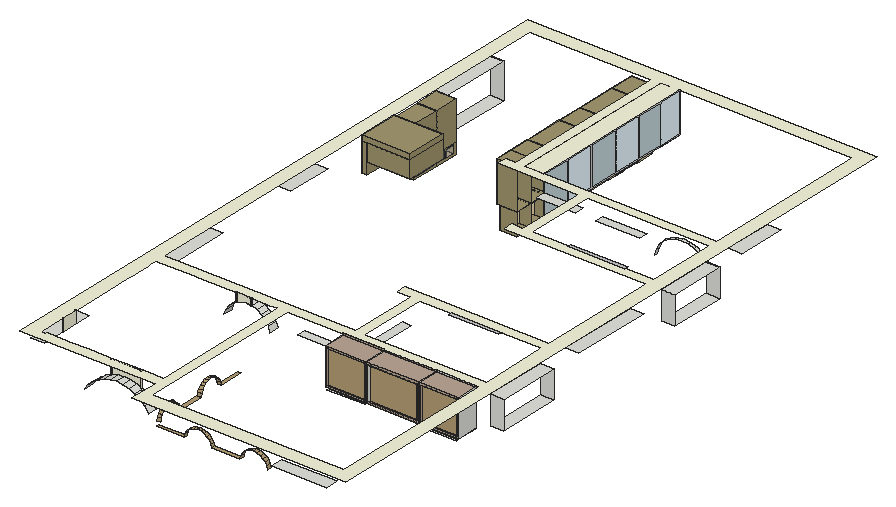
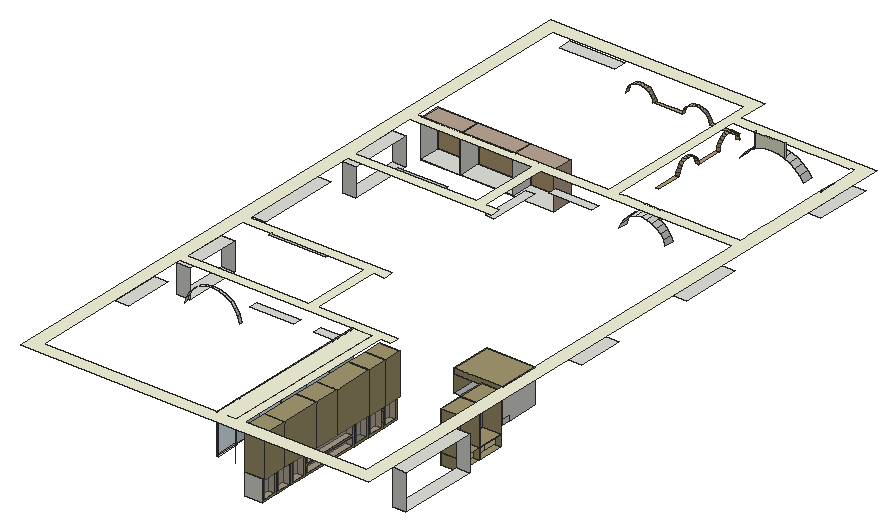
# SketchUp Ruby script. Lengths in inches.
U = 1.inch
M = Sketchup.active_model
def pt(a) = Geom::Point3d.new(a.map { |v| v * U })
def face(e, loops, mat)
  f = e.add_face(loops[0].map { |a| pt(a) })
  loops[1..].each { |l| e.add_face(l.map { |a| pt(a) }).erase! }
  f.material = f.back_material = mat if mat
  f
end
# faces: each face lists its corners as indices into pts; further lists are holes
def faces(e, pts, list, mat = nil) = list.each { |f| face(e, (f[0].is_a?(Array) ? f : [f]).map { |l| l.map { |i| pts[i] } }, mat) }
# xy, xz, yz: faces in a plane at the given z, y or x. An outline is a flat list of corners, or four numbers for a rectangle; further outlines are holes
def ring(l) = l.size == 4 ? [[l[0], l[1]], [l[2], l[1]], [l[2], l[3]], [l[0], l[3]]] : l.each_slice(2).to_a
def flat(e, list, mat, &to3) = list.each { |f| face(e, (f[0].is_a?(Array) ? f : [f]).map { |l| ring(l).map { |u, v| to3.(u, v) } }, mat) }
def xy(e, z, list, mat = nil) = flat(e, list, mat) { |x, y| [x, y, z] }
def xz(e, y, list, mat = nil) = flat(e, list, mat) { |x, z| [x, y, z] }
def yz(e, x, list, mat = nil) = flat(e, list, mat) { |y, z| [x, y, z] }
def lines(e, pts, list) = list.each { |a, b| e.add_line(pt(pts[a]), pt(pts[b])) }
# prism: a flat outline (further loops are holes) pulled along v
def prism(e, loops, v, mat = nil)
  f = face(e, loops, mat); d = Geom::Vector3d.new(v.map { |x| x * U })
  f.pushpull(f.normal.samedirection?(d) ? d.length : -d.length)
end
def box(e, o, s, mat = nil) = prism(e, [[o, [o[0] + s[0], o[1], o[2]], [o[0] + s[0], o[1] + s[1], o[2]], [o[0], o[1] + s[1], o[2]]]], [0, 0, s[2]], mat)
def at(x, y, z, deg = 0) = Geom::Transformation.translation(pt([x, y, z])) * Geom::Transformation.rotation(ORIGIN, Z_AXIS, deg.degrees)
def axes(o, x, y, z) = Geom::Transformation.new([*x, 0, *y, 0, *z, 0, *pt(o).to_a, 1])
def part(name) = M.definitions.add(name)
# library, detail: a bought-in or finely detailed component or shape, given as its bounding box
def library(name, o, s) = part(name).tap { |d| box(d.entities, o, s) }
def detail(e, o, s) = box(e.add_group.entities, o, s)
def put(e, d, t, mat = nil) = e.add_instance(d, t).tap { |i| i.material = mat if mat }
def group(e, t, mat = nil) = e.add_group.tap { |g| g.transformation = t; g.material = mat if mat }.entities
root = M.entities
M.materials.add("[0034_Wheat]").color = [245, 222, 179]
M.materials.add("[0049_Beige]").color = [245, 245, 220]
M.materials.add("[0093_AliceBlue]").color = [232, 248, 255]
M.materials.add("[0095_LightBlue]").color = [197, 216, 221]
M.materials.add("[0119_RosyBrown]").color = [188, 166, 148]
M.materials.add("[0132_LightGray]").color = [169, 169, 169]
M.materials.add("[Carrera Marble]").color = [207, 207, 207]
M.materials.add("[Ornate Tile 01]").color = [202, 202, 202]
M.materials.add("[Ornate Tile 02]").color = [201, 201, 201]
M.materials.add("[Translucent Glass Gray]").color = [128, 128, 128]
M.materials["[Translucent Glass Gray]"].alpha = 0.5
M.materials.add("[Wallpaper Thin Brown Stripes]").color = [182, 160, 118]
M.materials.add("[Wood Lumber ButtJoined]").color = [164, 152, 112]
xy(root,74.375,[[81.125,330.5,93,342.5],[81.125,342.99,93,354.99],[81.125,355.39,93,367.39],[81.125,367.79,93,409.3],[81.125,409.7,93,421.7],
  [81.125,422.1,93,434.1],[81.125,434.5,93,446.5]],"[Wood Lumber ButtJoined]")
xy(root,75.375,[[81.125,331.5,85.875,341.5],[81.125,343.99,85.875,353.99],[81.125,368.79,85.875,408.3],[81.125,410.7,85.875,420.7],[81.125,423.1,85.875,433.1],
  [81.125,435.5,85.875,445.5]],"[0034_Wheat]")
xy(root,75.375,[[81.125,356.39,85.875,366.39]],"[Wood Lumber ButtJoined]")
xy(root,81.08,[[81.125,368.79,85.875,408.3]],"[0034_Wheat]")
xy(root,81.8125,[[81.125,368.79,85.875,408.3]],"[0034_Wheat]")
xy(root,83.7,[[9,331.5,21.5,350.0625],[9,350.25,21.5,367.1875]],"[Wood Lumber ButtJoined]")
xy(root,84.7,[[12.5625,340.53,21.5,341.09],[12.5625,358.53,21.5,359.02]])
xy(root,84.7,[[12.5625,332.5,21.5,340.53],[12.5625,341.09,21.5,349.0625],[12.5625,351.25,21.5,358.53],[12.5625,359.02,21.5,366.1875]],"[0034_Wheat]")
xy(root,87.5625,[[0,369.625,9,424.25]])
xy(root,88.25,[[81.125,331.5,85.875,341.5],[81.125,343.99,85.875,353.99],[81.125,356.39,85.875,366.39],[81.125,368.79,85.875,408.3],[81.125,410.7,85.875,420.7],
  [81.125,423.1,85.875,433.1],[81.125,435.5,85.875,445.5]],"[0034_Wheat]")
xy(root,89.25,[[81.125,355.39,93,367.39],[81.125,367.79,93,409.3]])
xy(root,89.25,[[81.125,330.5,93,342.5],[81.125,342.99,93,354.99],[81.125,409.7,93,421.7],[81.125,422.1,93,434.1],[81.125,434.5,93,446.5]],"[Wood Lumber ButtJoined]")
xy(root,89.4375,[[79.125,330.5,93,342.84],[79.125,342.99,93,356.99],[79.125,357.2,93,384.45],[79.125,384.7,93,401.95],[79.125,402.1,93,429.35],
  [79.125,429.5,93,446.5]],"[Wood Lumber ButtJoined]")
xy(root,90.26,[[12.5625,332.5,21.5,340.53],[12.5625,341.09,21.5,349.0625],[12.5625,351.25,21.5,358.53],[12.5625,359.02,21.5,366.1875]],"[0034_Wheat]")
xy(root,91.26,[[9,331.5,21.5,350.0625],[9,350.25,21.5,367.1875]],"[Wood Lumber ButtJoined]")
xy(root,91.5625,[[9,331.5,22.125,350.0625],[9,350.25,22.125,367.1875]],"[Wood Lumber ButtJoined]")
xy(root,92,[[231,135.375,240,178.8125],[231,282.5625,240,321.125]])
xy(root,92.17,[[202.62,111,227.31,112.1875]])
xy(root,92.18,[[111.3125,350.49,112,370.8125],[111.3125,392.31,112,411.67],[111.3125,430.5,112,446.4]])
xy(root,92.2,[[138.21,111,163.85,112.1875]])
xy(root,93.18,[[111.5,330.5,112,350.375],[111.5,371.18,112,392.06],[111.5,411.92,112,430.3]],"[Carrera Marble]")
xy(root,93.41,[[137,111,165.0625,126],[165.15,111,201.29,126],[201.375,111,228.5625,126]])
xy(root,93.5625,[[137,111,165.0625,126],[165.15,111,201.29,126],[201.375,111,228.5625,126]])
xy(root,94.54,[[202.35,111,227.59,112.1875]],"[0119_RosyBrown]")
xy(root,94.64,[[138.08,111,163.98,112.1875]],"[0119_RosyBrown]")
xy(root,94.89,[[166.48,111,199.96,112.1875]],"[0119_RosyBrown]")
xy(root,96.5,[[9,302.05,12.875,330]])
xy(root,101.92,[[99,31.4,101.25,48.4],[99,66.3,101.25,83.1]],"[Wallpaper Thin Brown Stripes]")
xy(root,102.01,[[102.48,9,121.18,11.25],[140.76,9,159.46,11.25]],"[Wallpaper Thin Brown Stripes]")
xy(root,104.75,[[12.875,302.05,42.3125,330]],"[0132_LightGray]")
xy(root,108,[[105.75,126,136,132],[141,137.75,147,172.25],[112,324,138.73,330],[152.79,324,183.21,330]])
xy(root,111.25,[[231,135.375,240,178.8125],[231,200.3125,240,256],[231,282.5625,240,321.125],[231,340.4375,240,373.75]])
xy(root,111.6875,[[188.875,0,226.8125,9]])
xy(root,111.75,[[0,29.375,0,67.375,9.5,67.375,9.5,56.09,9,56.09,9,55.89,9.5,55.89,9.5,45.39,9,45.39,9,45.1875,9.25,45.1875,9.25,29.375],[0,141.25,9,183],[0,241.5625,9,273.5],[0,369.625,9,424.25]])
xy(root,113.91,[[64.01,125.5625,64.21,126]],"[0049_Beige]")
xy(root,116.5,[[9,302.05,12.875,330],[12.875,302.05,42.3125,330]])
xy(root,117.625,[[79.125,330.5,93,342.84],[79.125,342.99,93,356.99],[79.125,357.2,93,384.45],[79.125,384.7,93,401.95],[79.125,402.1,93,429.35],
  [79.125,429.5,93,446.5]],"[Wood Lumber ButtJoined]")
xy(root,117.67,[[166.48,111,199.96,112.1875]],"[0119_RosyBrown]")
xy(root,117.92,[[138.08,111,163.98,112.1875]],"[0119_RosyBrown]")
xy(root,118.02,[[202.35,111,227.59,112.1875]],"[0119_RosyBrown]")
xy(root,118.3125,[[9,331.5,22.125,350.0625],[9,350.25,22.125,367.1875]],"[Wood Lumber ButtJoined]")
xy(root,119,[[137,111,165.0625,126],[165.15,111,201.29,126],[201.375,111,228.5625,126]],"[0119_RosyBrown]")
xy(root,119.5,[[111.5,371.18,112,392.06],[111.5,411.92,112,430.3]])
xy(root,119.5,[[111.5,330.5,112,350.375]],"[Carrera Marble]")
xy(root,120,[[[93,0,240,0,240,456,0,456,0,20,93,20],[9,132,9,447,93,447,93,330,86,330,86,324,141,324,141,276,133.48,276,133.48,270,231,270,231,186,131.5,186,131.5,180,141,180,141,132],[99,9,231,126],[112,330,231,447],[9.25,26,9.25,45.1875,9,45.1875,9,45.39,9.5,45.39,9.5,55.89,9,55.89,9,56.09,9.5,56.09,9.5,71.78,9,71.78,9,71.98,9.5,71.98,9.5,83.1,9,83.1,9,83.3,9.5,83.3,9.5,102.55,9,102.55,9,102.75,9.5,102.75,9.5,118.43,9,118.43,9,125.5625,30.5625,125.5625,30.5625,126,30.76,126,30.76,125.5625,42.33,125.5625,42.33,126,42.53,126,42.53,125.5625,64.01,125.5625,64.01,126,64.21,126,64.21,125.5625,74.41,125.5625,74.41,126,74.6,126,74.6,125.5625,88.16,125.5625,88.16,126,93,126,93,26.8125,78.0625,26.8125,78.0625,26,77.86,26,77.86,26.8125,57.8,26.8125,57.8,26,57.6,26,57.6,26.8125,41.25,26.8125,41.25,26,41.05,26,41.05,26.8125,29.25,26.8125,29.25,26,29.05,26,29.05,26.8125,12.5625,26.8125,12.5625,26],[147,132,231,180],[147,276,231,324]]],"[0049_Beige]")
xy(root,120,[[168.74,177.6875,203.125,180]],"[Ornate Tile 01]")
xy(root,120,[[171.75,276,211.1875,278.4375]],"[Ornate Tile 02]")
xy(root,120,[[9,302.05,42.3125,330]],"[Wood Lumber ButtJoined]")
xz(root,26,[[57.6,110.54,57.8,110.63,57.8,110.54]])
xz(root,26,[[78.0625,109.3125,77.86,109.4,77.86,120,78.0625,120],[57.6,110.54,57.6,120,57.8,120,57.8,110.63]],"[0049_Beige]")
xz(root,26.8125,[[77.86,109.4,75,110.68,70.79,111.76,66.46,112.125,62.125,111.76,57.92,110.68,57.8,110.63,57.8,120,77.86,120]],"[0049_Beige]")
xz(root,45.1875,[[9,111.75,9.25,120]],"[0049_Beige]")
xz(root,45.39,[[9,111.75,9.5,120]],"[0049_Beige]")
xz(root,55.89,[[9,111.75,9.5,120]],"[0049_Beige]")
xz(root,56.09,[[9,111.75,9.5,120]],"[0049_Beige]")
xz(root,111,[[[137,93.5625,165.0625,119],[138.08,94.64,163.98,117.92]],[[165.15,93.5625,201.29,119],[166.48,94.89,199.96,117.67]],[[201.375,93.5625,228.5625,119],[202.35,94.54,227.59,118.02]]],"[0119_RosyBrown]")
xz(root,112.1875,[[202.35,94.54,227.59,118.02],[138.08,94.64,163.98,117.92],[166.48,94.89,199.96,117.67]],"[Wallpaper Thin Brown Stripes]")
xz(root,125.5625,[[64.21,113.91,64.54,114.11,67.96,115.29,71.5625,115.6875,74.41,115.37,74.41,120,64.21,120]],"[0049_Beige]")
xz(root,126,[[74.41,115.35,74.6,115.35,74.41,115.37],[201.6875,119,228.5625,120]])
xz(root,126,[[64.01,113.91,64.21,120],[74.6,115.35,74.6,120,74.41,120,74.41,115.37]],"[0049_Beige]")
xz(root,126,[[137,119,165.0625,120],[165.46,119,201.29,120]],"[0119_RosyBrown]")
xz(root,135.375,[[231,92,240,111.25]])
xz(root,178.8125,[[231,92,240,111.25]])
xz(root,282.5625,[[231,92,240,111.25]])
xz(root,302.05,[[9,96.5,12.875,116.5],[12.875,104.75,42.3125,116.5],[9,116.5,42.3125,120]],"[Wood Lumber ButtJoined]")
xz(root,321.125,[[231,92,240,111.25]])
xz(root,330,[[9,96.5,12.875,116.5],[9,116.5,42.3125,120]],"[Wood Lumber ButtJoined]")
xz(root,330.5,[[111.5,93.18,112,119.5]],"[Carrera Marble]")
xz(root,330.5,[[81.125,74.375,93,89.25],[79.125,89.4375,93,117.625]],"[Wood Lumber ButtJoined]")
xz(root,331.5,[[81.125,75.375,85.875,88.25]],"[0034_Wheat]")
xz(root,331.5,[[9,83.7,21.5,91.26],[9,91.5625,22.125,118.3125]],"[Wood Lumber ButtJoined]")
xz(root,332.5,[[12.5625,84.7,21.5,90.26]],"[0034_Wheat]")
xz(root,340.53,[[12.5625,84.7,21.5,90.26]],"[0034_Wheat]")
xz(root,341.09,[[12.5625,84.7,21.5,90.26]],"[0034_Wheat]")
xz(root,341.5,[[81.125,75.375,85.875,88.25]],"[0034_Wheat]")
xz(root,342.5,[[81.125,74.375,93,89.25]],"[Wood Lumber ButtJoined]")
xz(root,342.84,[[79.125,89.4375,93,117.625]],"[Wood Lumber ButtJoined]")
xz(root,342.99,[[81.125,74.375,93,89.25],[79.125,89.4375,93,117.625]],"[Wood Lumber ButtJoined]")
xz(root,343.99,[[81.125,75.375,85.875,88.25]],"[0034_Wheat]")
xz(root,349.0625,[[12.5625,84.7,21.5,90.26]],"[0034_Wheat]")
xz(root,350.0625,[[9,83.7,21.5,91.26],[9,91.5625,22.125,118.3125]],"[Wood Lumber ButtJoined]")
xz(root,350.25,[[9,83.7,21.5,91.26],[9,91.5625,22.125,118.3125]],"[Wood Lumber ButtJoined]")
xz(root,350.375,[[111.5,93.18,112,119.5]],"[Carrera Marble]")
xz(root,351.25,[[12.5625,84.7,21.5,90.26]],"[0034_Wheat]")
xz(root,353.99,[[81.125,75.375,85.875,88.25]],"[0034_Wheat]")
xz(root,354.99,[[81.125,74.375,93,89.25]],"[Wood Lumber ButtJoined]")
xz(root,355.39,[[81.125,74.375,93,89.25]],"[Wood Lumber ButtJoined]")
xz(root,356.39,[[81.125,75.375,85.875,88.25]],"[0034_Wheat]")
xz(root,356.99,[[79.125,89.4375,93,117.625]],"[Wood Lumber ButtJoined]")
xz(root,357.2,[[79.125,89.4375,93,117.625]],"[Wood Lumber ButtJoined]")
xz(root,358.53,[[12.5625,84.7,21.5,90.26]],"[0034_Wheat]")
xz(root,359.02,[[12.5625,84.7,21.5,90.26]],"[0034_Wheat]")
xz(root,366.1875,[[12.5625,84.7,21.5,90.26]],"[0034_Wheat]")
xz(root,366.39,[[81.125,75.375,85.875,88.25]],"[0034_Wheat]")
xz(root,367.1875,[[9,83.7,21.5,91.26],[9,91.5625,22.125,118.3125]],"[Wood Lumber ButtJoined]")
xz(root,367.39,[[81.125,74.375,93,89.25]],"[Wood Lumber ButtJoined]")
xz(root,367.79,[[81.125,74.375,93,89.25]],"[Wood Lumber ButtJoined]")
xz(root,368.79,[[81.125,81.08,85.875,81.8125]])
xz(root,368.79,[[81.125,75.375,85.875,81.08],[81.125,81.8125,85.875,88.25]],"[0034_Wheat]")
xz(root,369.625,[[0,87.5625,9,111.75]])
xz(root,371.18,[[111.5,93.18,112,119.5]])
xz(root,384.45,[[79.125,89.4375,93,117.625]],"[Wood Lumber ButtJoined]")
xz(root,384.7,[[79.125,89.4375,93,117.625]],"[Wood Lumber ButtJoined]")
xz(root,392.06,[[111.5,93.18,112,119.5]],"[Carrera Marble]")
xz(root,401.95,[[79.125,89.4375,93,117.625]],"[Wood Lumber ButtJoined]")
xz(root,402.1,[[79.125,89.4375,93,117.625]],"[Wood Lumber ButtJoined]")
xz(root,408.3,[[81.125,75.375,85.875,81.08],[81.125,81.8125,85.875,88.25]],"[0034_Wheat]")
xz(root,409.3,[[81.125,74.375,93,89.25]],"[Wood Lumber ButtJoined]")
xz(root,409.7,[[81.125,74.375,93,89.25]],"[Wood Lumber ButtJoined]")
xz(root,410.7,[[81.125,75.375,85.875,88.25]],"[0034_Wheat]")
xz(root,411.92,[[111.5,93.18,112,119.5]])
xz(root,420.7,[[81.125,75.375,85.875,88.25]],"[0034_Wheat]")
xz(root,421.7,[[81.125,74.375,93,89.25]],"[Wood Lumber ButtJoined]")
xz(root,422.1,[[81.125,74.375,93,89.25]],"[Wood Lumber ButtJoined]")
xz(root,423.1,[[81.125,75.375,85.875,88.25]],"[0034_Wheat]")
xz(root,424.25,[[0,87.5625,9,111.75]])
xz(root,429.35,[[79.125,89.4375,93,117.625]],"[Wood Lumber ButtJoined]")
xz(root,429.5,[[79.125,89.4375,93,117.625]],"[Wood Lumber ButtJoined]")
xz(root,430.3,[[111.5,93.18,112,119.5]],"[Carrera Marble]")
xz(root,433.1,[[81.125,75.375,85.875,88.25]],"[0034_Wheat]")
xz(root,434.1,[[81.125,74.375,93,89.25]],"[Wood Lumber ButtJoined]")
xz(root,434.5,[[81.125,74.375,93,89.25]],"[Wood Lumber ButtJoined]")
xz(root,435.5,[[81.125,75.375,85.875,88.25]],"[0034_Wheat]")
xz(root,445.5,[[81.125,75.375,85.875,88.25]],"[0034_Wheat]")
xz(root,446.5,[[81.125,74.375,93,89.25]])
xz(root,446.5,[[79.125,89.4375,93,117.625]],"[Wood Lumber ButtJoined]")
xz(root,447,[[111.3125,92.68,112,120]])
yz(root,9,[[302.05,96.5,302.05,116.5,330,116.5,330,100.1875,324,100.1875,324,96.5],[324,96.5,330,100.1875]])
yz(root,9,[[45.1875,111.75,45.39,120],[55.89,111.75,56.09,120]],"[0049_Beige]")
yz(root,9,[[302.05,116.5,330,120]],"[0132_LightGray]")
yz(root,9.5,[[45.39,111.75,55.89,120]],"[0049_Beige]")
yz(root,12.5625,[[332.5,84.7,340.53,90.26],[341.09,84.7,349.0625,90.26],[351.25,84.7,358.53,90.26],[359.02,84.7,366.1875,90.26]],"[0034_Wheat]")
yz(root,12.875,[[302.05,96.5,324,104.75],[324,96.5,330,104.75],[302.05,104.75,330,116.5]],"[Wood Lumber ButtJoined]")
yz(root,21.5,[[332.5,84.7,340.53,90.26],[341.09,84.7,349.0625,90.26],[351.25,84.7,358.53,90.26],[359.02,84.7,366.1875,90.26]],"[Translucent Glass Gray]")
yz(root,21.5,[[[331.5,83.7,350.0625,91.26],[332.5,84.7,340.53,90.26],[341.09,84.7,349.0625,90.26]],[[350.25,83.7,367.1875,91.26],[351.25,84.7,358.53,90.26],[359.02,84.7,366.1875,90.26]]],"[Wood Lumber ButtJoined]")
yz(root,22.125,[[331.5,91.5625,350.0625,118.3125],[350.25,91.5625,367.1875,118.3125]],"[Wood Lumber ButtJoined]")
yz(root,42.3125,[[302.05,104.75,330,116.5],[302.05,116.5,330,120]],"[Wood Lumber ButtJoined]")
yz(root,57.6,[[26,110.54,26.8125,120]],"[0049_Beige]")
yz(root,57.8,[[26,110.63,26.8125,120]],"[0049_Beige]")
yz(root,64.01,[[125.5625,113.91,126,120]],"[0049_Beige]")
yz(root,64.21,[[125.5625,113.91,126,120]],"[0049_Beige]")
yz(root,74.41,[[125.5625,115.37,126,120]],"[0049_Beige]")
yz(root,74.6,[[125.5625,115.35,126,120]],"[0049_Beige]")
yz(root,77.86,[[26,109.4,26.8125,120]],"[0049_Beige]")
yz(root,78.0625,[[26,109.3125,26.8125,120]],"[0049_Beige]")
yz(root,79.125,[[330.5,89.4375,342.84,117.625],[342.99,89.4375,356.99,117.625],[357.2,89.4375,384.45,117.625],[384.7,89.4375,401.95,117.625],[402.1,89.4375,429.35,117.625],
  [429.5,89.4375,446.5,117.625]],"[Wood Lumber ButtJoined]")
yz(root,81.125,[[331.5,75.375,341.5,88.25],[343.99,75.375,353.99,88.25],[356.39,75.375,366.39,88.25],[368.79,75.375,408.3,81.08],[410.7,75.375,420.7,88.25],
  [423.1,75.375,433.1,88.25],[435.5,75.375,445.5,88.25],[368.79,81.8125,408.3,88.25]],"[Translucent Glass Gray]")
yz(root,81.125,[[[330.5,74.375,342.5,89.25],[331.5,75.375,341.5,88.25]],[[342.99,74.375,354.99,89.25],[343.99,75.375,353.99,88.25]],[[355.39,74.375,367.39,89.25],[356.39,75.375,366.39,88.25]],[[367.79,74.375,409.3,89.25],[368.79,81.8125,408.3,88.25],[368.79,75.375,408.3,81.08]],[[409.7,74.375,421.7,89.25],[410.7,75.375,420.7,88.25]],
  [[422.1,74.375,434.1,89.25],[423.1,75.375,433.1,88.25]],[[434.5,74.375,446.5,89.25],[435.5,75.375,445.5,88.25]]],"[Wood Lumber ButtJoined]")
yz(root,85.875,[[331.5,75.375,341.5,88.25],[343.99,75.375,353.99,88.25],[356.39,75.375,366.39,88.25],[368.79,75.375,408.3,81.08],[410.7,75.375,420.7,88.25],
  [423.1,75.375,433.1,88.25],[435.5,75.375,445.5,88.25],[368.79,81.8125,408.3,88.25]],"[0034_Wheat]")
yz(root,111.5,[[330.5,93.18,350.375,119.5],[371.18,93.18,392.06,119.5],[411.92,93.18,430.3,119.5]],"[0095_LightBlue]")
yz(root,112,[[350.58,93.18,370.88,119.5],[392.26,93.18,411.625,119.5],[430.5,93.18,446.5,119.5]],"[0093_AliceBlue]")
yz(root,112,[[[330,92.68,447,120],[371.18,93.18,392.06,119.5],[350.58,93.18,370.88,119.5],[330.5,93.18,350.375,119.5],[392.26,93.18,411.625,119.5],[411.92,93.18,430.3,119.5],[430.5,93.18,446.5,119.5]]],"[Carrera Marble]")
yz(root,137,[[111,93.5625,126,119]],"[0119_RosyBrown]")
yz(root,138.08,[[111,94.64,112.1875,117.92]],"[0119_RosyBrown]")
yz(root,163.98,[[111,94.64,112.1875,117.92]],"[0119_RosyBrown]")
yz(root,165.0625,[[111,93.5625,126,119]])
yz(root,165.15,[[111,93.5625,126,119]])
yz(root,166.48,[[111,94.89,112.1875,117.67]])
yz(root,199.96,[[111,94.89,112.1875,117.67]],"[0119_RosyBrown]")
yz(root,201.29,[[111,93.5625,126,119]])
yz(root,201.375,[[111,93.5625,126,119]])
yz(root,202.35,[[111,94.54,112.1875,118.02]],"[0119_RosyBrown]")
yz(root,227.59,[[111,94.54,112.1875,118.02]],"[0119_RosyBrown]")
yz(root,228.5625,[[111,93.5625,126,119]])
p = [[188.21,330,96.52],[189.51,330,100.76],[189.51,331.8125,100.76],[188.21,331.8125,96.52],[224.7,330,100.76],[226,330,96.52],
  [226,331.8125,96.52],[224.7,331.8125,100.76],[47.16,20,103.53],[44.53,20,100.0625],[44.53,26.8125,100.0625],[47.16,26.8125,103.53],
  [88.38,20,100.0625],[85.75,20,103.53],[85.75,26,103.53],[88.38,26,100.0625],[85.75,26.8125,103.53],[88.38,26.8125,100.0625],
  [191.75,330,104.6],[191.75,331.8125,104.6],[222.46,330,104.6],[222.46,331.8125,104.6],[99,14.37,104.05],[99,14,101.92],
  [101.1875,14,101.92],[101.1875,14.37,104.05],[99,31,101.92],[99,30.63,104.05],[101.1875,30.63,104.05],[101.1875,31,101.92],
  [99,49.17,104.05],[99,48.8,101.92],[101.25,48.8,101.92],[101.25,49.17,104.05],[99,65.8,101.92],[99,65.43,104.05],
  [101.25,65.43,104.05],[101.25,65.8,101.92],[121.62,9,102.01],[122.05,9,104.12],[122.05,11.25,104.12],[121.62,11.25,102.01],
  [139.89,9,104.12],[140.32,9,102.01],[140.32,11.25,102.01],[139.89,11.25,104.12],[160.12,9,102.01],[160.54,9,104.125],
  [160.54,11.75,104.125],[160.12,11.75,102.01],[178.4,9,104.125],[178.82,9,102.01],[178.82,11.75,102.01],[178.4,11.75,104.125],
  [56.89,132,106.64],[56.89,125.5625,106.64],[55.625,125.5625,103.25],[55.625,132,103.25],[87.5,132,103.25],[87.5,125.5625,103.25],
  [86.24,125.5625,106.64],[86.24,132,106.64],[50.33,20,106.5],[50.33,26.8125,106.5],[82.59,20,106.5],[82.59,26,106.5],
  [82.59,26.8125,106.5],[99,15.27,106.01],[101.1875,15.27,106.01],[99,29.73,106.01],[101.1875,29.73,106.01],[99,50.07,106.01],
  [101.25,50.07,106.01],[99,64.53,106.01],[101.25,64.53,106.01],[123.04,9,106.06],[123.04,11.25,106.06],[138.89,9,106.06],
  [138.89,11.25,106.06],[161.53,9,106.08],[161.53,11.75,106.08],[177.41,9,106.08],[177.41,11.75,106.08],[194.81,330,107.8125],
  [194.81,331.8125,107.8125],[219.41,330,107.8125],[219.41,331.8125,107.8125],[99,16.625,107.6875],[101.1875,16.625,107.6875],[99,28.375,107.6875],
  [101.1875,28.375,107.6875],[99,51.42,107.6875],[101.25,51.42,107.6875],[99,63.18,107.6875],[101.25,63.18,107.6875],[124.54,9,107.71],
  [124.54,11.25,107.71],[137.4,9,107.71],[137.4,11.25,107.71],[163.03,9,107.74],[163.03,11.75,107.74],[175.91,9,107.74],
  [175.91,11.75,107.74],[53.95,20,108.91],[53.95,26.8125,108.91],[78.97,20,108.91],[78.97,26,108.91],[78.97,26.8125,108.91],
  [58.86,132,109.68],[58.86,125.5625,109.68],[84.26,125.5625,109.68],[84.26,132,109.68],[126.44,9,108.98],[126.44,11.25,108.98],
  [135.49,9,108.98],[135.49,11.25,108.98],[164.93,9,109.01],[164.93,11.75,109.01],[174.01,9,109.01],[174.01,11.75,109.01],
  [99,18.36,108.97],[101.1875,18.36,108.97],[99,26.64,108.97],[101.1875,26.64,108.97],[99,53.16,108.97],[101.25,53.16,108.97],
  [99,61.44,108.97],[101.25,61.44,108.97],[198.52,330,110.24],[198.52,331.8125,110.24],[215.69,330,110.24],[215.69,331.8125,110.24],
  [57.92,20,110.68],[57.6,26.8125,110.54],[57.6,26,110.54],[57.8,26,110.63],[57.8,26.8125,110.63],[57.92,26.8125,110.68],
  [75,20,110.68],[75,26.8125,110.68],[77.86,26.8125,109.4],[77.86,26,109.4],[78.0625,26,109.3125],[78.0625,26.8125,109.3125],
  [128.63,9,109.77],[128.63,11.25,109.77],[133.31,9,109.77],[133.31,11.25,109.77],[167.125,9,109.8],[167.125,11.75,109.8],
  [171.8125,9,109.8],[171.8125,11.75,109.8],[99,20.36,109.77],[101.1875,20.36,109.77],[99,24.64,109.77],[101.1875,24.64,109.77],
  [99,55.16,109.77],[101.25,55.16,109.77],[99,59.4375,109.77],[101.25,59.4375,109.77],[61.45,132,112.21],[61.45,125.5625,112.21],
  [81.67,125.5625,112.21],[81.67,132,112.21],[130.97,9,110.04],[130.97,11.25,110.04],[169.47,9,110.08],[169.47,11.75,110.08],
  [99,22.5,110.04],[101.1875,22.5,110.04],[99,57.3,110.04],[101.25,57.3,110.04],[202.7,330,111.75],[202.7,331.8125,111.75],
  [211.52,330,111.75],[211.52,331.8125,111.75],[62.125,20,111.76],[62.125,26.8125,111.76],[70.79,20,111.76],[70.79,26.8125,111.76],
  [66.46,20,112.125],[66.46,26.8125,112.125],[207.11,330,112.27],[207.11,331.8125,112.27],[64.54,132,114.11],[64.54,125.5625,114.11],
  [64.21,125.5625,113.91],[78.59,125.5625,114.11],[78.59,132,114.11],[67.96,132,115.29],[67.96,125.5625,115.29],[75.16,125.5625,115.29],
  [75.16,132,115.29],[71.5625,132,115.6875],[71.5625,125.5625,115.6875],[74.6,126,115.35],[74.41,126,115.37],[74.41,125.5625,115.37],
  [74.6,125.5625,115.35],[9,302.05,120],[9,302.05,120.29],[99,447,120],[104.6875,447,120],[99,447,92.68],
  [99,330,120],[112,330,120]]
faces(root,p,[[0,1,2,3],[4,5,6,7],[8,9,10,11],[12,13,14,15],[1,18,19,2],[20,4,7,21],[54,55,56,57],[58,59,60,61],
  [62,8,11,63],[13,64,65,14],[18,83,84,19],[85,20,21,86],[103,62,63,104],[64,105,106,65],[108,109,55,54],[61,60,110,111],
  [83,128,129,84],[130,85,86,131],[132,103,104,133,134,135,136,137],[105,138,139,140,141,142,106],[160,161,109,108],[111,110,162,163],[128,172,173,129],[174,130,131,175],
  [176,132,137,177],[138,178,179,139],[180,176,177,181],[178,180,181,179],[172,182,183,173],[182,174,175,183],[184,185,186,161,160],[163,162,187,188],
  [189,190,185,184],[188,187,191,192],[193,194,190,189],[195,196,197,194,193,192,191,198]])
faces(root,p,[[15,14,16,17],[14,65,66,16],[65,106,107,66],[106,142,143,107]],"[0049_Beige]")
faces(root,p,[[22,23,24,25],[26,27,28,29],[30,31,32,33],[34,35,36,37],[38,39,40,41],[42,43,44,45],[46,47,48,49],[50,51,52,53],
  [67,22,25,68],[27,69,70,28],[71,30,33,72],[35,73,74,36],[39,75,76,40],[77,42,45,78],[47,79,80,48],[81,50,53,82],
  [87,67,68,88],[69,89,90,70],[91,71,72,92],[73,93,94,74],[75,95,96,76],[97,77,78,98],[79,99,100,80],[101,81,82,102],
  [95,112,113,96],[114,97,98,115],[99,116,117,100],[118,101,102,119],[120,87,88,121],[89,122,123,90],[124,91,92,125],[93,126,127,94],
  [112,144,145,113],[146,114,115,147],[116,148,149,117],[150,118,119,151],[152,120,121,153],[122,154,155,123],[156,124,125,157],[126,158,159,127],
  [144,164,165,145],[164,146,147,165],[148,166,167,149],[166,150,151,167],[168,152,153,169],[154,168,169,155],[170,156,157,171],[158,170,171,159]],"[Wallpaper Thin Brown Stripes]")
lines(root,p,[[199,200],[201,202],[203,201],[204,201],[205,204]])
